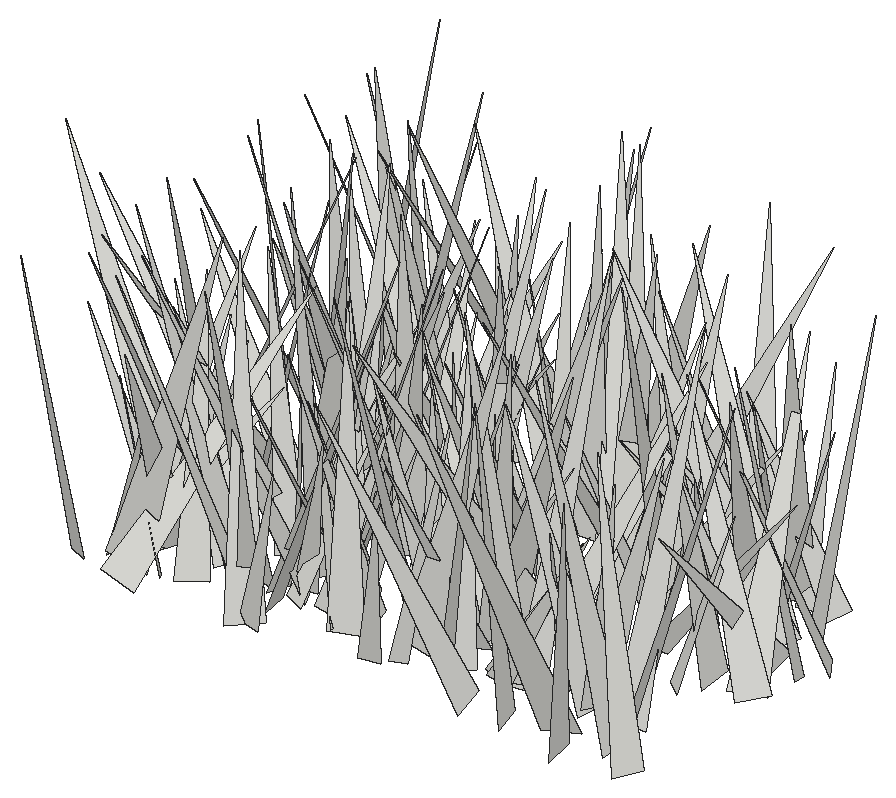
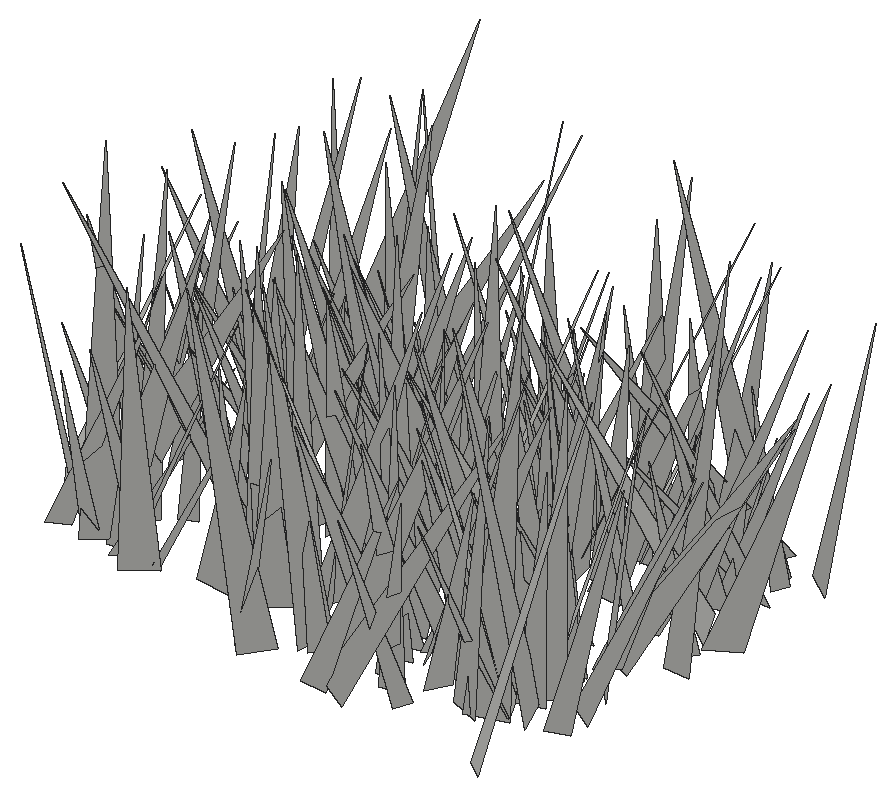
# SketchUp Ruby script. Lengths in inches.
U = 1.inch
M = Sketchup.active_model
def pt(a) = Geom::Point3d.new(a.map { |v| v * U })
def face(e, loops, mat)
  f = e.add_face(loops[0].map { |a| pt(a) })
  loops[1..].each { |l| e.add_face(l.map { |a| pt(a) }).erase! }
  f.material = f.back_material = mat if mat
  f
end
# faces: each face lists its corners as indices into pts; further lists are holes
def faces(e, pts, list, mat = nil) = list.each { |f| face(e, (f[0].is_a?(Array) ? f : [f]).map { |l| l.map { |i| pts[i] } }, mat) }
# xy, xz, yz: faces in a plane at the given z, y or x. An outline is a flat list of corners, or four numbers for a rectangle; further outlines are holes
def ring(l) = l.size == 4 ? [[l[0], l[1]], [l[2], l[1]], [l[2], l[3]], [l[0], l[3]]] : l.each_slice(2).to_a
def flat(e, list, mat, &to3) = list.each { |f| face(e, (f[0].is_a?(Array) ? f : [f]).map { |l| ring(l).map { |u, v| to3.(u, v) } }, mat) }
def xy(e, z, list, mat = nil) = flat(e, list, mat) { |x, y| [x, y, z] }
def xz(e, y, list, mat = nil) = flat(e, list, mat) { |x, z| [x, y, z] }
def yz(e, x, list, mat = nil) = flat(e, list, mat) { |y, z| [x, y, z] }
def lines(e, pts, list) = list.each { |a, b| e.add_line(pt(pts[a]), pt(pts[b])) }
# prism: a flat outline (further loops are holes) pulled along v
def prism(e, loops, v, mat = nil)
  f = face(e, loops, mat); d = Geom::Vector3d.new(v.map { |x| x * U })
  f.pushpull(f.normal.samedirection?(d) ? d.length : -d.length)
end
def box(e, o, s, mat = nil) = prism(e, [[o, [o[0] + s[0], o[1], o[2]], [o[0] + s[0], o[1] + s[1], o[2]], [o[0], o[1] + s[1], o[2]]]], [0, 0, s[2]], mat)
def at(x, y, z, deg = 0) = Geom::Transformation.translation(pt([x, y, z])) * Geom::Transformation.rotation(ORIGIN, Z_AXIS, deg.degrees)
def axes(o, x, y, z) = Geom::Transformation.new([*x, 0, *y, 0, *z, 0, *pt(o).to_a, 1])
def part(name) = M.definitions.add(name)
# library, detail: a bought-in or finely detailed component or shape, given as its bounding box
def library(name, o, s) = part(name).tap { |d| box(d.entities, o, s) }
def detail(e, o, s) = box(e.add_group.entities, o, s)
def put(e, d, t, mat = nil) = e.add_instance(d, t).tap { |i| i.material = mat if mat }
def group(e, t, mat = nil) = e.add_group.tap { |g| g.transformation = t; g.material = mat if mat }.entities
root = M.entities
c1 = part("fur_instance\#9")
p = [[0.8125,0,1.79],[0.67,-0.02,1.48],[0,-0.11,0],[0,0.11,0]]
faces(c1.entities,p,[[0,1,2,3]])
put(root,c1,axes([86.87,12.82,-27.1],[0.82289,-7.98079,0.80674],[-7.83354,-0.97405,-1.64552],[-1.72608,0.61581,7.85254]))
put(root,c1,axes([82.93,12.35,-27.1],[-6.88482,-1.0416,0.48285],[-0.90858,6.73783,1.57954],[0.70182,-1.49517,6.78165]))
put(root,c1,axes([87.8,11.51,-27.1],[5.74214,0.07937,1.80023],[0.34922,-5.94743,-0.85168],[-1.76782,-0.91707,5.67918]))
put(root,c1,axes([73.07,11.85,-27.1],[0.44262,-3.83329,1.02735],[-3.85493,-0.16968,1.02773],[0.94293,1.1057,3.71938]))
put(root,c1,axes([72.28,12.92,-27.1],[3.06057,-3.28635,0.3748],[-3.27189,-3.08287,-0.31361],[-0.4851,0.05914,4.47983]))
put(root,c1,axes([78.15,12.54,-27.1],[1.46502,-3.697,0.60293],[-3.73698,-1.39797,0.50827],[0.25762,0.74531,3.94408]))
put(root,c1,axes([84.83,12.2,-27.1],[-6.1633,-1.76581,2.36846],[-1.74431,6.59751,0.37966],[2.38433,0.26209,6.40002]))
put(root,c1,axes([64.88,12.16,-27.1],[-3.28868,-4.79968,1.75844],[-5.10998,3.14053,-0.98472],[0.13097,2.01112,5.73434]))
put(root,c1,axes([72.51,12.72,-27.1],[-6.31151,-2.93767,0.11387],[-2.9284,6.25835,-0.85765],[-0.25951,0.82534,6.90866]))
put(root,c1,axes([67.33,14.95,-27.1],[4.65411,-4.15615,0.09318],[-4.0063,-4.52139,-1.56511],[-1.10988,-1.10744,6.04026]))
put(root,c1,axes([80.74,13.75,-27.1],[4.65665,4.64477,2.8893],[5.46904,-4.02795,-2.33914],[-0.10763,-3.71592,6.14709]))
put(root,c1,axes([66.7,12.73,-27.1],[0.11593,7.32982,3.76994],[7.80213,1.11829,-2.4142],[2.6581,-3.60212,6.9218]))
put(root,c1,axes([65.85,13.19,-27.1],[3.70802,-0.97097,0.29213],[-0.94384,-3.70994,-0.3508],[-0.37053,-0.26665,3.81695]))
put(root,c1,axes([90.75,11.82,-27.1],[-5.69821,2.17721,0.97614],[2.15034,5.78116,-0.34192],[1.034,-0.02439,6.0904]))
put(root,c1,axes([71.31,14.75,-27.1],[-1.28259,-7.19659,1.19017],[-7.23451,1.40948,0.72639],[0.93233,1.03678,7.27381]))
put(root,c1,axes([72.92,11.83,-27.1],[-5.4488,4.52209,1.619],[4.59694,5.6194,-0.22458],[1.39234,-0.85616,7.07731]))
put(root,c1,axes([89.22,13.1,-27.1],[-7.32255,-0.11088,1.35528],[-0.08815,7.44603,0.13288],[1.35695,-0.11461,7.32218]))
put(root,c1,axes([68.26,12.73,-27.1],[-3.16034,-1.96863,0.75138],[-2.10046,2.8354,-1.40585],[-0.16774,1.5852,3.44773]))
put(root,c1,axes([73.25,15.2,-27.1],[-6.90561,-3.33755,0.10935],[-3.32242,6.89219,0.54573],[0.33571,-0.44394,7.65042]))
put(root,c1,axes([77.89,15.62,-27.1],[-6.44031,-4.10602,1.97316],[-3.85542,6.73281,1.42663],[2.42663,-0.20036,7.50344]))
put(root,c1,axes([86.81,14.86,-27.1],[-6.00437,2.1113,1.91932],[2.55574,5.96789,1.43049],[1.26869,-2.0299,6.20191]))
put(root,c1,axes([82.78,14.26,-27.1],[1.91277,-3.82749,0.78831],[-3.61325,-1.39793,1.9799],[1.48846,1.5251,3.7932]))
put(root,c1,axes([76.21,13.58,-27.1],[-2.20554,5.93145,2.00046],[6.2413,2.24627,0.22087],[0.47966,-1.95462,6.32437]))
put(root,c1,axes([78.94,14.35,-27.1],[1.45839,-7.20301,2.88114],[-7.56056,-0.66269,2.17028],[1.73849,3.16049,7.02141]))
put(root,c1,axes([80.76,15.79,-27.1],[-0.13118,-4.53208,0.33432],[-4.41868,0.04908,-1.06843],[-1.06148,0.35576,4.40629]))
put(root,c1,axes([71.19,13.97,-27.1],[-7.48937,-0.81173,0.36322],[-0.84224,7.4632,-0.68756],[0.28542,0.72333,7.50179]))
put(root,c1,axes([73.09,15.18,-27.1],[1.90373,-3.64825,0.45227],[-3.65968,-1.83258,0.622],[0.34793,0.68584,4.0678]))
put(root,c1,axes([69.4,13.125,-27.1],[-4.06626,4.25963,1.22614],[4.27905,4.20638,-0.4224],[1.15655,-0.5867,5.87371]))
put(root,c1,axes([76.52,15.16,-27.1],[-5.39834,-1.72938,0.70035],[-1.70183,5.44274,0.32197],[0.76486,-0.09564,5.65943]))
put(root,c1,axes([84.68,15.7,-27.1],[-1.23844,-4.00226,0.78585],[-3.84524,1.41955,1.16979],[1.36007,0.36904,4.02286]))
put(root,c1,axes([67.08,14.8,-27.1],[-4.89818,0.93846,0.55806],[1.01529,4.8584,0.74127],[0.40164,-0.83642,4.93188]))
put(root,c1,axes([82.5,14.49,-27.1],[1.50617,-3.93782,1.16858],[-3.70084,-0.76096,2.20573],[1.78207,1.74788,3.59301]))
put(root,c1,axes([83.39,14.53,-27.1],[0.00148,-6.83986,3.17541],[-7.42007,-0.56775,-1.21947],[-1.34516,3.12424,6.73027]))
put(root,c1,axes([74.7,15.98,-27.1],[-2.68226,-4.58353,0.12394],[-4.53778,2.63294,-0.83358],[-0.65781,0.52677,5.24485]))
put(root,c1,axes([72.86,13.58,-27.1],[6.72772,1.76518,0.89994],[1.69777,-6.77807,0.60273],[-1.02144,0.36032,6.92927]))
put(root,c1,axes([67.28,11.46,-27.1],[-1.44675,6.62808,0.1342],[5.91861,1.35324,-3.03008],[2.98656,0.529,6.06986]))
put(root,c1,axes([86.77,14.86,-27.1],[4.38951,-2.01268,1.547],[-2.15257,-4.58905,0.13732],[-1.34555,0.7756,4.82698]))
put(root,c1,axes([74.67,14.4,-27.1],[-0.11814,4.24138,1.60816],[4.31681,0.59918,-1.26317],[1.39308,-1.49704,4.05064]))
put(root,c1,axes([75.74,13.76,-27.1],[-4.50739,-0.00087,0.31518],[-0.09503,4.31184,-1.34718],[0.30051,1.35052,4.30136]))
put(root,c1,axes([79.03,13.12,-27.1],[-4.41847,1.33903,1.10997],[0.76139,4.21375,-2.05244],[1.56375,1.73183,4.13562]))
put(root,c1,axes([67.36,16.77,-27.1],[-2.8111,-5.64649,0.53318],[-5.64839,2.7334,-0.83291],[-0.51273,0.84565,6.25232]))
put(root,c1,axes([82.77,17.87,-27.1],[1.75618,-7.20882,1.45322],[-6.25973,-2.24953,-3.59425],[-3.85938,0.3683,6.49097]))
put(root,c1,axes([73.26,14.25,-27.1],[1.23248,3.89294,0.26564],[3.83774,-1.15903,-0.82034],[0.70519,-0.49622,4.00013]))
put(root,c1,axes([78.68,15.93,-27.1],[-5.18821,0.426,1.12668],[0.56814,5.25845,0.62796],[1.06213,-0.73187,5.16766]))
put(root,c1,axes([81.22,13.99,-27.1],[-5.70691,2.72816,1.15825],[2.57005,5.80682,-1.01437],[1.47624,0.43731,6.24361]))
put(root,c1,axes([69.62,15.03,-27.1],[-4.99004,2.24313,0.58277],[2.2784,5.00139,0.2583],[0.42444,-0.4756,5.46492]))
put(root,c1,axes([75.4375,16.54,-27.1],[-3.54687,-2.63553,0.56126],[-2.61948,3.58991,0.30355],[0.63194,0.08835,4.40842]))
put(root,c1,axes([66.41,13.9375,-27.1],[-0.23722,4.19444,0.05409],[3.55446,0.22976,-2.22834],[2.22756,0.08005,3.56147]))
put(root,c1,axes([68.89,15.07,-27.1],[-3.32365,-1.7064,1.24939],[-2.04417,3.18881,-1.08271],[0.54234,1.56176,3.57578]))
put(root,c1,axes([70.47,17.6875,-27.1],[2.04194,-5.37013,1.21962],[-4.97283,-2.35693,-2.05211],[-2.36574,0.31918,5.36625]))
put(root,c1,axes([75.47,15.28,-27.1],[3.08965,-1.86478,1.07968],[-2.12915,-2.93231,1.02827],[-0.33144,1.45368,3.45919]))
put(root,c1,axes([80.73,16.62,-27.1],[5.91489,-2.56905,1.81184],[-2.61095,-6.16477,-0.21752],[-1.75092,0.51416,6.44505]))
put(root,c1,axes([80.55,17.06,-27.1],[5.68552,-4.38043,0.51347],[-4.40819,-5.61738,0.88871],[0.14016,1.01677,7.12204]))
put(root,c1,axes([71.83,16.22,-27.1],[1.95949,2.80373,1.45551],[3.04239,-2.136,0.01872],[-0.85045,-1.18135,3.42055]))
put(root,c1,axes([66.7,15.77,-27.1],[1.07751,-3.9043,2.33703],[-4.53898,-0.75293,0.83488],[0.32078,2.46086,3.96327]))
put(root,c1,axes([72.22,14.65,-27.1],[6.79493,0.95964,1.40947],[0.56386,-6.72962,1.86359],[-1.60922,1.6941,6.60447]))
put(root,c1,axes([72.9,16.36,-27.1],[4.01633,-1.15722,1.23996],[-1.33038,-4.12648,0.45808],[-1.05202,0.80037,4.15454]))
put(root,c1,axes([65.91,14.4375,-27.1],[1.29367,6.30142,0.29631],[6.29029,-1.26564,-0.54746],[0.47747,-0.39942,6.4095]))
put(root,c1,axes([88.75,14.47,-27.1],[5.94248,2.0649,1.47313],[1.51819,-5.90154,2.14801],[-2.032,1.62942,5.91295]))
put(root,c1,axes([88.48,14.72,-27.1],[0.44326,7.59594,0.73525],[7.62112,-0.4789,0.35297],[-0.39679,-0.71255,7.60067]))
put(root,c1,axes([73.14,16.7,-27.1],[6.72571,2.73267,0.89443],[2.78268,-6.75899,-0.27437],[-0.72399,-0.59256,7.25447]))
put(root,c1,axes([79.02,17.53,-27.1],[3.3459,3.39415,0.39754],[3.18536,-2.89609,-2.08314],[1.23764,-1.72213,4.2867]))
put(root,c1,axes([77.96,15.9,-27.1],[5.23362,2.8594,0.35445],[2.818,-5.23298,0.60609],[-0.60055,0.36375,5.93293]))
put(root,c1,axes([81.11,16.67,-27.1],[-3.6214,4.75768,0.36392],[4.63089,3.39426,1.70771],[-1.15013,-1.31374,5.73008]))
put(root,c1,axes([80.07,19.28,-27.1],[0.31088,-6.10314,0.84199],[-6.04835,-0.46277,-1.12122],[-1.17245,0.76905,6.00731]))
put(root,c1,axes([71.03,16.88,-27.1],[-1.86081,5.49202,1.44787],[5.66351,1.67938,0.90859],[-0.42807,-1.65488,5.72707]))
put(root,c1,axes([77.08,17.72,-27.1],[4.20297,-1.11156,0.80651],[-1.18233,-4.24977,0.30429],[-0.69867,0.5049,4.33681]))
put(root,c1,axes([84.1,14.4,-27.1],[1.42623,8.08681,0.06748],[7.92603,-1.41139,1.61901],[-1.60595,0.21606,8.05043]))
put(root,c1,axes([64.93,20.38,-27.1],[-2.27672,-7.40144,1.23154],[-7.29478,2.48469,1.44709],[1.75622,0.72557,7.60728]))
put(root,c1,axes([75.4375,19.6,-27.1],[-5.5722,-4.07145,0.43281],[-4.071,5.58734,0.1482],[0.43699,0.13539,6.89957]))
put(root,c1,axes([76.88,18.14,-27.1],[4.42426,3.38365,0.88099],[3.49585,-4.30744,-1.01209],[-0.06566,-1.34021,5.47712]))
put(root,c1,axes([64.62,18.07,-27.1],[-5.80896,4.38047,0.69826],[4.41604,5.60261,1.59041],[-0.41794,-1.68592,7.09952]))
put(root,c1,axes([76.01,18.44,-27.1],[-2.1087,-2.96786,0.97974],[-3.12443,1.97245,-0.74971],[-0.07759,1.23123,3.56269]))
put(root,c1,axes([72.08,17.23,-27.1],[-6.95078,-0.2098,1.40903],[-0.48679,6.94525,-1.36721],[1.33881,1.43604,6.81821]))
put(root,c1,axes([89.95,21.74,-27.1],[4.40481,-2.70951,0.82389],[-1.71706,-3.76665,-3.20728],[-2.2521,-2.42766,4.05674]))
put(root,c1,axes([88.07,17.87,-27.1],[2.28219,3.09258,0.57784],[3.14608,-2.24088,-0.43237],[0.01087,-0.72161,3.81909]))
put(root,c1,axes([88.875,19.24,-27.1],[-6.33484,-0.15602,2.15214],[0.09289,6.64883,0.75543],[2.15578,-0.74496,6.29157]))
put(root,c1,axes([80.07,20.8,-27.1],[-0.6438,-6.00502,0.1729],[-5.98541,0.62626,-0.53591],[-0.51472,0.22839,6.0156]))
put(root,c1,axes([67.98,18.71,-27.1],[-5.05806,4.73106,0.08976],[4.36112,4.60989,2.7757],[-1.83619,-2.08349,6.34527]))
put(root,c1,axes([65.36,19.125,-27.1],[1.8239,-3.22944,0.77362],[-3.28665,-1.6292,0.94764],[0.47508,1.1273,3.58579]))
put(root,c1,axes([77.46,18.54,-27.1],[-4.422,-0.95671,1.75223],[-1.16644,4.69405,-0.38074],[1.6202,0.76828,4.50826]))
put(root,c1,axes([79.42,18.2,-27.1],[2.90611,1.79436,1.69144],[1.585,-3.36196,0.84331],[-1.88904,-0.06039,3.30969]))
put(root,c1,axes([74.49,19.61,-27.1],[2.05152,-6.96349,2.48946],[-7.36809,-2.14532,0.07104],[-0.63146,2.40909,7.25905]))
put(root,c1,axes([72.55,19.59,-27.1],[3.14021,-1.95272,0.11029],[-1.95573,-3.13292,0.21476],[0.01996,0.24059,3.6916]))
put(root,c1,axes([73.45,20.54,-27.1],[0.26156,-6.27199,1.2943],[-6.21893,0.06053,1.55008],[1.52905,1.31908,6.08306]))
put(root,c1,axes([75.52,19.56,-27.1],[2.21811,-2.97156,1.30139],[-3.14682,-2.35396,-0.01147],[-0.78819,1.03561,3.7081]))
put(root,c1,axes([67.13,21.23,-27.1],[-0.73144,-5.99959,0.26703],[-5.39662,0.53861,-2.681],[-2.63493,0.56233,5.41685]))
put(root,c1,axes([89.89,20.37,-27.1],[-4.18916,1.41328,1.44955],[1.84035,4.04661,1.3732],[0.84361,-1.80976,4.20247]))
put(root,c1,axes([84,19.54,-27.1],[1.31447,-3.85278,1.5031],[-4.0825,-0.95693,1.11736],[0.66058,1.75255,3.91449]))
put(root,c1,axes([70.5,19.84,-27.1],[2.46707,-3.42013,1.11602],[-3.59628,-2.30764,0.87798],[0.09798,1.4166,4.12467]))
put(root,c1,axes([71.97,19.35,-27.1],[2.76185,-3.07557,2.49035],[-3.57907,-3.23702,-0.02845],[-1.68858,1.83068,4.13354]))
put(root,c1,axes([90.82,19.0625,-27.1],[-3.78677,4.88862,0.77178],[4.90876,3.58599,1.37062],[-0.63111,-1.44081,6.0299]))
put(root,c1,axes([72.1875,20.54,-27.1],[2.06201,-3.51619,0.27094],[-3.44771,-1.94389,1.0117],[0.74186,0.73932,3.94867]))
put(root,c1,axes([65.99,17.14,-27.1],[6.85876,3.23862,0.41321],[3.02392,-6.66397,2.03701],[-1.23097,1.67477,7.30628]))
put(root,c1,axes([77.49,18.74,-27.1],[5.50822,-3.47682,2.75588],[-4.25576,-5.38219,1.71589],[-1.25366,2.99458,6.28367]))
put(root,c1,axes([67.02,20.01,-27.1],[6.14666,2.4589,1.36982],[2.59506,-6.2248,-0.47069],[-1.09008,-0.95377,6.60349]))
put(root,c1,axes([83.87,21.76,-27.1],[-4.5248,-1.88356,0.71077],[-1.69814,4.51006,1.14127],[1.08134,-0.799,4.76646]))
put(root,c1,axes([85.78,19.74,-27.1],[3.92135,-2.35365,0.03406],[-2.05535,-3.39138,2.27856],[1.14733,1.96892,3.96545]))
put(root,c1,axes([77.99,17.03,-27.1],[-7.05102,3.6652,1.50452],[2.87345,6.84526,-3.20935],[2.72774,2.26338,7.26985]))
put(root,c1,axes([75.72,18.65,-27.1],[-0.62554,4.99616,0.12365],[4.99768,0.62512,0.02455],[-0.009,-0.12574,5.03511]))
put(root,c1,axes([83.17,22.34,-27.1],[-1.63485,-6.2778,0.46595],[-5.97391,1.39539,-2.16005],[-1.98499,0.97094,6.117]))
put(root,c1,axes([81.95,18.95,-27.1],[1.01067,5.88602,0.15693],[5.68933,-0.93518,-1.56469],[1.51703,-0.41415,5.76354]))
put(root,c1,axes([70.53,21.48,-27.1],[4.49175,-3.99144,0.42922],[-3.97143,-4.32409,1.3497],[0.58618,1.28931,5.8554]))
put(root,c1,axes([76.25,22.36,-27.1],[6.0824,-3.06076,1.36011],[-2.97573,-6.23245,-0.71791],[-1.53726,-0.04598,6.77115]))
put(root,c1,axes([83.47,23.09,-27.1],[-6.68782,-2.79113,3.18251],[-2.04813,7.34131,2.13449],[3.70459,-0.98003,6.92541]))
put(root,c1,axes([68.82,24.1,-27.1],[1.6119,-7.35068,0.1441],[-7.34568,-1.61634,-0.28263],[-0.30696,0.08011,7.52003]))
put(root,c1,axes([85.86,22.63,-27.1],[0.30074,-4.21199,0.28121],[-4.14735,-0.24225,0.80695],[0.78703,0.33293,4.14489]))
put(root,c1,axes([74.26,24.16,-27.1],[4.06405,-3.6671,0.18626],[-3.28339,-3.75381,-2.26428],[-1.64366,-1.56845,4.98369]))
put(root,c1,axes([91.61,22.58,-27.1],[-5.39414,-3.77764,0.22745],[-3.78403,5.38986,-0.22257],[0.05845,0.31282,6.58162]))
put(root,c1,axes([87.12,23.62,-27.1],[6.03542,-2.39463,0.80521],[-2.12324,-5.9379,-1.74415],[-1.3691,-1.34759,6.25448]))
put(root,c1,axes([84.47,21.91,-27.1],[3.53808,2.09554,0.91862],[2.27584,-3.39762,-1.01485],[-0.23603,-1.34836,3.98489]))
put(root,c1,axes([72.92,18.65,-27.1],[5.4592,3.52611,0.65952],[3.05756,-5.20187,2.50265],[-1.87611,1.78282,5.99776]))
put(root,c1,axes([68.83,20.67,-27.1],[1.67584,3.97009,0.12724],[3.80521,-1.56498,-1.28741],[1.13936,-0.61275,4.1125]))
put(root,c1,axes([77.63,21.77,-27.1],[2.98572,-5.88102,1.99527],[-6.13329,-2.44486,1.97166],[0.97482,2.63026,6.29392]))
put(root,c1,axes([81.78,19.36,-27.1],[-2.11402,4.56513,0.60738],[3.84978,2.11854,-2.52378],[2.52756,0.59144,4.35202]))
put(root,c1,axes([67.08,21.72,-27.1],[-4.48303,2.72425,0.35571],[2.72908,4.33728,1.17718],[-0.3165,-1.18832,5.11208]))
put(root,c1,axes([67.66,23.03,-27.1],[0.9975,-5.62203,0.93729],[-5.55991,-0.75041,1.41599],[1.25425,1.14473,5.53148]))
put(root,c1,axes([90.42,19.18,-27.1],[-4.33285,5.33033,0.39838],[5.19442,4.31986,-1.30443],[1.26061,0.52067,6.74422]))
put(root,c1,axes([72.56,21.54,-27.1],[3.74419,-3.98525,0.35569],[-3.51637,-3.04515,2.89653],[1.90889,2.20738,4.63803]))
put(root,c1,axes([81.13,19.44,-27.1],[-6.61706,2.95045,0.41304],[2.75432,6.44194,-1.89112],[1.13554,1.56763,6.99387]))
put(root,c1,axes([91.19,21.26,-27.1],[-5.46466,-2.11839,0.66349],[-2.21236,5.05235,-2.09036],[-0.18243,2.18553,5.47545]))
put(root,c1,axes([77.83,21.05,-27.1],[6.41211,-0.61612,1.30158],[-0.93497,-6.2989,1.62436],[-1.09524,1.77006,6.23347]))
put(root,c1,axes([70.88,20.59,-27.1],[-0.70792,6.63222,0.94241],[6.69223,0.65809,0.39581],[-0.29764,-0.97786,6.65814]))
put(root,c1,axes([77.05,22.83,-27.1],[-4.90354,-1.85753,0.89414],[-1.8937,4.97041,-0.05944],[0.81474,0.37312,5.24324]))
put(root,c1,axes([83.23,22.2,-27.1],[3.04424,4.32162,0.01521],[3.85535,-2.70735,-2.39804],[1.95268,-1.39208,4.71097]))
put(root,c1,axes([89.12,22.68,-27.1],[-4.49913,6.58347,1.21187],[6.27218,3.63575,3.53468],[-2.33889,-2.91414,7.14775]))
put(root,c1,axes([81.84,21.23,-27.1],[0.68062,5.93772,0.86921],[5.89172,-0.495,-1.23203],[1.14003,-0.98679,5.84823]))
put(root,c1,axes([67.07,23.62,-27.1],[6.76883,1.43904,1.95286],[1.74836,-6.90673,-0.9705],[-1.68159,-1.38844,6.85171]))
put(root,c1,axes([73.89,21.14,-27.1],[-1.59492,4.69203,0.53683],[4.53057,1.68008,-1.22409],[1.33316,-0.09626,4.80214]))
put(root,c1,axes([68.02,23.87,-27.1],[-5.59539,-3.44886,0.89561],[-3.54081,5.56848,-0.67808],[0.39927,1.05,6.53783]))
put(root,c1,axes([76.33,23.94,-27.1],[-3.68845,0.83243,0.84341],[0.99836,3.66829,0.74556],[0.6384,-0.92717,3.70698]))
put(root,c1,axes([84.67,25.94,-27.1],[-4.21387,-1.59887,0.24339],[-1.27519,3.70248,2.24451],[0.99474,-2.02671,3.90836]))
put(root,c1,axes([83.42,22.4,-27.1],[-1.23701,6.48468,1.94316],[6.59867,1.59608,-1.12573],[1.51147,-1.6609,6.50492]))
put(root,c1,axes([86.75,25.79,-27.1],[-1.94792,-5.41513,0.85515],[-5.11405,2.12183,1.78705],[1.97517,0.15336,5.47032]))
put(root,c1,axes([66.1875,23.02,-27.1],[-4.69579,-3.74143,2.09942],[-4.25802,4.44495,-1.60248],[0.52452,2.58851,5.78625]))
put(root,c1,axes([65.65,25.07,-27.1],[-2.53227,-4.93937,0.36335],[-4.86121,2.40071,-1.24381],[-0.94765,0.88376,5.4095]))
put(root,c1,axes([87.44,25.6875,-27.1],[4.02071,-6.30995,0.86141],[-6.36147,-4.02715,0.19326],[-0.29869,0.83076,7.47959]))
put(root,c1,axes([88.56,22.97,-27.1],[4.03699,1.00135,1.00845],[0.75439,-4.0837,1.03503],[-1.2044,0.79854,4.02849]))
put(root,c1,axes([77.62,24.77,-27.1],[-4.6895,-2.45579,1.69505],[-2.43913,4.97359,0.45768],[1.71894,0.35769,5.27378]))
put(root,c1,axes([88.63,23.15,-27.1],[-6.09178,4.42452,0.24879],[4.41982,6.03543,0.88707],[-0.32169,-0.86331,7.47659]))
put(root,c1,axes([86.35,26.29,-27.1],[-4.14982,-0.72477,0.23143],[-0.53834,3.70403,1.94686],[0.53763,-1.88541,3.73578]))
put(root,c1,axes([82.15,24.47,-27.1],[-3.43259,1.11019,2.13702],[1.24058,4.00441,-0.08763],[2.06406,-0.56053,3.60659]))
put(root,c1,axes([67.32,24.87,-27.1],[-4.56803,3.68378,2.77525],[4.20348,4.93276,0.37129],[1.89817,-2.05836,5.85656]))
put(root,c1,axes([68.46,24.05,-27.1],[2.21445,2.95218,0.72503],[3.03203,-2.20951,-0.26401],[-0.21871,-0.73996,3.68096]))
put(root,c1,axes([70.8,25.78,-27.1],[0.6809,-4.24063,0.83858],[-4.19337,-0.85411,-0.91428],[-1.04966,0.66131,4.19651]))
put(root,c1,axes([82.3125,22.92,-27.1],[2.96543,7.80813,0.73471],[7.53088,-2.61577,-2.59693],[2.18919,-1.57838,7.9383]))
put(root,c1,axes([65.54,26.56,-27.1],[3.46395,-3.11936,0.86631],[-2.7787,-3.51575,-1.54862],[-1.66124,-0.62369,4.39672]))
put(root,c1,axes([79.36,25.65,-27.1],[2.15737,-6.51602,1.69287],[-6.69271,-1.88316,1.28061],[0.7294,1.99342,6.74336]))
put(root,c1,axes([78.76,24.61,-27.1],[-0.16128,6.84934,2.86842],[7.42417,0.20732,-0.07764],[0.15166,-2.86546,6.8508]))
put(root,c1,axes([72.83,22.67,-27.1],[-4.26385,3.34064,0.29483],[3.15748,4.15963,-1.468],[1.13011,0.98225,5.21395]))
put(root,c1,axes([89.44,25.73,-27.1],[-4.32688,2.05759,1.06704],[2.30248,4.07514,1.47851],[0.2661,-1.80382,4.55737]))
put(root,c1,axes([78.07,24.29,-27.1],[-7.19785,3.45896,0.52945],[3.49375,7.17168,0.64382],[0.19618,-0.81015,7.95983]))
put(root,c1,axes([70.93,22.49,-27.1],[7.1916,2.06862,2.54607],[1.20326,-7.37063,2.58975],[-3.05186,1.96861,7.0208]))
put(root,c1,axes([86.28,24.84,-27.1],[3.72364,-1.08643,0.80362],[-1.21362,-3.72465,0.58799],[-0.59435,0.79892,3.83407]))
put(root,c1,axes([72.51,24.55,-27.1],[-5.71185,4.45959,0.23835],[4.39877,5.55102,1.55146],[-0.77178,-1.36683,7.07857]))
put(root,c1,axes([73.46,25.88,-27.1],[0.07384,-6.03784,2.03973],[-6.28438,0.27016,1.02718],[1.05955,2.02311,5.95028]))
put(root,c1,axes([86.18,25.46,-27.1],[-5.88175,-1.50758,0.15009],[-1.51502,5.85044,-0.60606],[-0.00586,0.62434,6.04156]))
put(root,c1,axes([72.93,24.53,-27.1],[-7.75285,-2.01113,0.68817],[-2.11722,7.53738,-1.82488],[0.1887,1.94117,7.79879]))
put(root,c1,axes([80.83,24.35,-27.1],[-1.87564,7.62096,1.95831],[7.8685,1.80971,0.49369],[-0.027,-2.0194,7.83284]))
put(root,c1,axes([68.62,25.03,-27.1],[4.54931,-2.96003,1.24819],[-3.21199,-4.22741,1.68171],[-0.05363,2.09362,5.16041]))
put(root,c1,axes([71.14,25.07,-27.1],[0.71966,5.69009,1.64056],[5.43341,0.02279,-2.46251],[2.35511,-1.79132,5.17987]))
put(root,c1,axes([76.89,23.32,-27.1],[-5.00496,1.9066,1.35129],[1.19771,4.83542,-2.3864],[2.00664,1.8693,4.79477]))
put(root,c1,axes([77.54,22.6875,-27.1],[5.51307,6.12337,0.96272],[5.81555,-5.55551,2.03274],[-2.14519,0.67601,7.98483]))
put(root,c1,axes([67.55,25.59,-27.1],[1.73924,-4.25815,2.51532],[-4.74882,-2.1825,-0.41111],[-1.38108,2.14207,4.58125]))
put(root,c1,axes([89.47,24.45,-27.1],[3.26782,5.25044,1.3347],[5.28581,-3.43164,0.55786],[-1.18691,-0.82697,6.1591]))
put(root,c1,axes([80.45,24.23,-27.1],[-5.1988,6.07272,1.14347],[6.1224,5.26442,-0.12263],[0.83765,-0.78798,7.99315]))
put(root,c1,axes([68.25,27.3,-27.1],[2.83404,-7.21043,2.36501],[-7.48804,-3.06648,-0.37599],[-1.22999,2.05469,7.73827]))
put(root,c1,axes([74.44,28.53,-27.1],[-0.7633,-7.78268,1.04828],[-7.63293,0.4877,-1.93706],[-1.84592,1.20152,7.57632]))
put(root,c1,axes([72.22,27.84,-27.1],[-0.22733,-5.68785,1.31588],[-5.73337,0.46581,1.02292],[1.10075,1.2515,5.59972]))
put(root,c1,axes([76.11,27.18,-27.1],[3.13443,-2.25979,0.73802],[-2.32723,-3.16608,0.18952],[-0.4851,0.5876,3.85946]))
put(root,c1,axes([67.9375,26.1,-27.1],[5.69643,3.12279,1.00252],[3.16084,-5.76326,-0.00802],[-0.87518,-0.48903,6.49623]))
put(root,c1,axes([88.14,25.48,-27.1],[0.35019,4.61175,0.40741],[4.56098,-0.41379,0.76359],[-0.79477,-0.34263,4.56155]))
put(root,c1,axes([73.7,25.05,-27.1],[-2.14385,5.53708,0.23418],[5.53457,2.15208,-0.21752],[0.2875,-0.13964,5.93364]))
put(root,c1,axes([82.11,25.93,-27.1],[-1.56415,5.71782,0.81541],[5.62888,1.31989,1.54221],[-1.29382,-1.17019,5.72377]))
put(root,c1,axes([76.65,26.76,-27.1],[7.07212,-1.1156,2.41076],[-1.38462,-7.39913,0.63784],[-2.26697,1.03896,7.1311]))
put(root,c1,axes([69.17,27.42,-27.1],[1.62899,5.48386,2.82302],[6.01922,-2.05055,0.50999],[-1.34582,-2.53344,5.69792]))
put(root,c1,axes([71.02,26.63,-27.1],[-4.64621,2.31988,0.55706],[2.32982,4.67441,-0.03457],[0.51391,-0.21773,5.19306]))
put(root,c1,axes([73.86,29.32,-27.1],[-2.5504,-6.61055,0.06946],[-6.29815,2.40698,-2.17909],[-2.00934,0.84606,6.74207]))
put(root,c1,axes([67.83,26.91,-27.1],[1.33461,3.80482,0.72121],[3.71713,-1.04467,-1.36733],[1.08616,-1.09999,3.79319]))
put(root,c1,axes([67.06,26.08,-27.1],[7.33246,2.99097,2.42144],[2.72494,-7.71469,1.27771],[-2.71735,0.33456,7.81527]))
put(root,c1,axes([66.19,30.57,-27.1],[-4.76858,-5.56642,0.65425],[-5.40433,4.79429,1.40014],[1.48534,-0.42682,7.19472]))
put(root,c1,axes([84.95,26.64,-27.1],[-3.82919,5.78151,1.38736],[5.88668,3.91838,-0.08139],[0.83523,-1.11076,6.93412]))
put(root,c1,axes([72.9,27.22,-27.1],[-1.18349,4.29439,0.91251],[4.36217,1.04349,0.74676],[-0.49586,-1.06979,4.39144]))
put(root,c1,axes([77.81,28.68,-27.1],[4.01839,-5.64573,1.18023],[-5.73753,-3.76564,1.52164],[0.58986,1.83314,6.76065]))
put(root,c1,axes([74.61,29.42,-27.1],[1.33499,-4.14938,1.03511],[-3.92508,-1.61935,-1.42916],[-1.69781,0.48101,4.1179]))
put(root,c1,axes([78.79,28.33,-27.1],[-3.8802,0.07929,1.10053],[0.11582,4.03064,0.11798],[1.09728,-0.14508,3.87922]))
put(root,c1,axes([71.18,28.49,-27.1],[2.09245,-2.98815,0.44058],[-2.87886,-1.81085,1.39087],[0.91397,1.13723,3.37237]))
